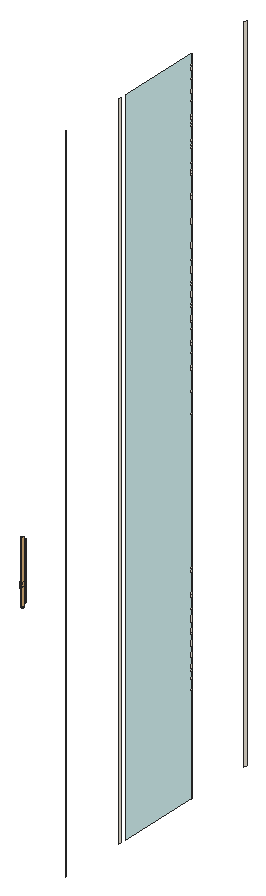
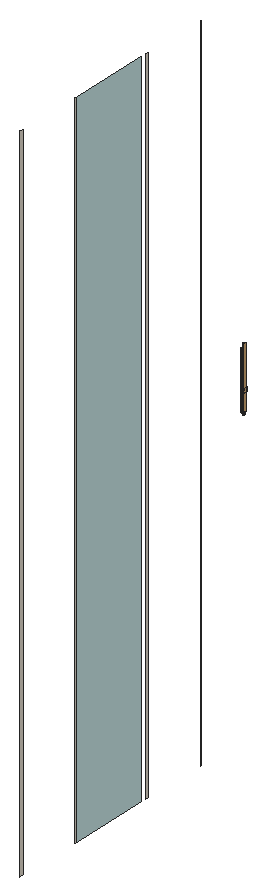
# SketchUp Ruby script. Lengths in inches.
U = 1.inch
M = Sketchup.active_model
def pt(a) = Geom::Point3d.new(a.map { |v| v * U })
def face(e, loops, mat)
  f = e.add_face(loops[0].map { |a| pt(a) })
  loops[1..].each { |l| e.add_face(l.map { |a| pt(a) }).erase! }
  f.material = f.back_material = mat if mat
  f
end
# faces: each face lists its corners as indices into pts; further lists are holes
def faces(e, pts, list, mat = nil) = list.each { |f| face(e, (f[0].is_a?(Array) ? f : [f]).map { |l| l.map { |i| pts[i] } }, mat) }
# xy, xz, yz: faces in a plane at the given z, y or x. An outline is a flat list of corners, or four numbers for a rectangle; further outlines are holes
def ring(l) = l.size == 4 ? [[l[0], l[1]], [l[2], l[1]], [l[2], l[3]], [l[0], l[3]]] : l.each_slice(2).to_a
def flat(e, list, mat, &to3) = list.each { |f| face(e, (f[0].is_a?(Array) ? f : [f]).map { |l| ring(l).map { |u, v| to3.(u, v) } }, mat) }
def xy(e, z, list, mat = nil) = flat(e, list, mat) { |x, y| [x, y, z] }
def xz(e, y, list, mat = nil) = flat(e, list, mat) { |x, z| [x, y, z] }
def yz(e, x, list, mat = nil) = flat(e, list, mat) { |y, z| [x, y, z] }
def lines(e, pts, list) = list.each { |a, b| e.add_line(pt(pts[a]), pt(pts[b])) }
# prism: a flat outline (further loops are holes) pulled along v
def prism(e, loops, v, mat = nil)
  f = face(e, loops, mat); d = Geom::Vector3d.new(v.map { |x| x * U })
  f.pushpull(f.normal.samedirection?(d) ? d.length : -d.length)
end
def box(e, o, s, mat = nil) = prism(e, [[o, [o[0] + s[0], o[1], o[2]], [o[0] + s[0], o[1] + s[1], o[2]], [o[0], o[1] + s[1], o[2]]]], [0, 0, s[2]], mat)
def at(x, y, z, deg = 0) = Geom::Transformation.translation(pt([x, y, z])) * Geom::Transformation.rotation(ORIGIN, Z_AXIS, deg.degrees)
def axes(o, x, y, z) = Geom::Transformation.new([*x, 0, *y, 0, *z, 0, *pt(o).to_a, 1])
def part(name) = M.definitions.add(name)
# library, detail: a bought-in or finely detailed component or shape, given as its bounding box
def library(name, o, s) = part(name).tap { |d| box(d.entities, o, s) }
def detail(e, o, s) = box(e.add_group.entities, o, s)
def put(e, d, t, mat = nil) = e.add_instance(d, t).tap { |i| i.material = mat if mat }
def group(e, t, mat = nil) = e.add_group.tap { |g| g.transformation = t; g.material = mat if mat }.entities
root = M.entities
M.materials.add("Material \#1").color = [140, 140, 140]
M.materials.add("[0030_OldLace]").color = [253, 245, 230]
M.materials.add("[0090_LightCyan]").color = [224, 255, 255]
c1 = library("3DGeom~1_Defintion",[-60.87,347.29,-704.08],[121.74,121.75,1000])
c2 = library("3DGeom~14_Defintion",[-102.17,352.37,-727.27],[204.35,204.35,1000])
c3 = part("3DGeom~5_Defintion")
xy(c3.entities,-225.24,[[-0.79,-499.98,-2.33,-499.64,7.45,-496.14],[-0.79,-499.98,7.45,-496.14,1.58,-499.88],[1.58,-499.88,7.45,-496.14,3.84,-499.16],[-2.33,-499.64,7.4,-485.75,7.45,-496.14],[3.84,-499.16,7.45,-496.14,5.85,-497.89],
  [7.45,-496.14,7.4,-485.75,8.24,-487.08],[7.45,-496.14,8.24,-487.08,8.96,-489.34],[7.45,-496.14,8.96,-489.34,9.0625,-491.71],[7.45,-496.14,9.0625,-491.71,8.55,-494.03],[-7.4,-496.08,-8.24,-494.76,2.32,-482.2],
  [-8.24,-494.76,-8.96,-492.5,2.32,-482.2],[-8.96,-492.5,-9.0625,-490.125,2.32,-482.2],[-9.0625,-490.125,-8.55,-487.81,2.32,-482.2],[-8.55,-487.81,-7.45,-485.7,2.32,-482.2],[-7.45,-485.7,-5.85,-483.95,2.32,-482.2],
  [-5.85,-483.95,-3.84,-482.68,2.32,-482.2],[-3.84,-482.68,-1.58,-481.96,2.32,-482.2],[2.32,-482.2,-1.58,-481.96,0.79,-481.86],[0,481.82,-2.35,482.13,-6.92,496.71],[0,481.82,-6.92,496.71,1.55,482.04],
  [-2.35,482.13,-4.55,483.04,-6.92,496.71],[-4.55,483.04,-6.43,484.49,-6.92,496.71],[-6.43,484.49,-7.88,486.37,-6.92,496.71],[6.92,485.12,-1.55,499.8125,7.88,495.47],[6.92,485.12,7.88,495.47,7.88,486.37],
  [-7.88,486.37,-8.79,488.57,-6.92,496.71],[7.88,486.37,7.88,495.47,8.79,488.57],[-8.79,488.57,-9.1,490.92,-6.92,496.71],[8.79,488.57,7.88,495.47,9.1,490.92],[-9.1,490.92,-8.79,493.28,-6.92,496.71],
  [9.1,490.92,7.88,495.47,8.79,493.28],[-8.79,493.28,-7.88,495.47,-6.92,496.71],[7.88,495.47,-1.55,499.8125,0,500.02],[7.88,495.47,0,500.02,2.35,499.71],[7.88,495.47,2.35,499.71,4.55,498.8],
  [7.88,495.47,4.55,498.8,6.43,497.35]],"Material \#1")
xy(c3.entities,-221.57,[[-2.33,-499.64,-5.22,-498.37,7.4,-485.75],[-5.22,-498.37,-7.4,-496.08,5.22,-483.47],[-5.22,-498.37,5.22,-483.47,7.4,-485.75],[-7.4,-496.08,2.32,-482.2,5.22,-483.47],[1.55,482.04,-6.92,496.71,-4.55,498.8],
  [1.55,482.04,-4.55,498.8,4.55,483.04],[4.55,483.04,-4.55,498.8,-1.55,499.8125],[4.55,483.04,-1.55,499.8125,6.92,485.12]],"Material \#1")
xy(c3.entities,38.05,[[-2.33,-499.64,7.4,-485.75,-5.22,-498.37],[-5.22,-498.37,5.22,-483.47,-7.4,-496.08],[-5.22,-498.37,7.4,-485.75,5.22,-483.47],[-7.4,-496.08,5.22,-483.47,2.32,-482.2],[1.55,482.04,-4.55,498.8,-6.92,496.71],
  [1.55,482.04,4.55,483.04,-4.55,498.8],[4.55,483.04,-1.55,499.8125,-4.55,498.8],[4.55,483.04,6.92,485.12,-1.55,499.8125]],"Material \#1")
xy(c3.entities,41.72,[[-0.79,-499.98,7.45,-496.14,-2.33,-499.64],[-0.79,-499.98,1.58,-499.88,7.45,-496.14],[1.58,-499.88,3.84,-499.16,7.45,-496.14],[-2.33,-499.64,7.45,-496.14,7.4,-485.75],[3.84,-499.16,5.85,-497.89,7.45,-496.14],
  [7.45,-496.14,8.24,-487.08,7.4,-485.75],[7.45,-496.14,8.55,-494.03,9.0625,-491.71],[7.45,-496.14,8.96,-489.34,8.24,-487.08],[7.45,-496.14,9.0625,-491.71,8.96,-489.34],[-7.4,-496.08,2.32,-482.2,-8.24,-494.76],
  [-8.24,-494.76,2.32,-482.2,-8.96,-492.5],[-8.96,-492.5,2.32,-482.2,-9.0625,-490.125],[-9.0625,-490.125,2.32,-482.2,-8.55,-487.81],[-8.55,-487.81,2.32,-482.2,-7.45,-485.7],[-7.45,-485.7,2.32,-482.2,-5.85,-483.95],
  [-5.85,-483.95,2.32,-482.2,-3.84,-482.68],[-3.84,-482.68,2.32,-482.2,-1.58,-481.96],[2.32,-482.2,0.79,-481.86,-1.58,-481.96],[0,481.82,-6.92,496.71,-2.35,482.13],[0,481.82,1.55,482.04,-6.92,496.71],
  [-2.35,482.13,-6.92,496.71,-4.55,483.04],[-4.55,483.04,-6.92,496.71,-6.43,484.49],[-6.43,484.49,-6.92,496.71,-7.88,486.37],[6.92,485.12,7.88,495.47,-1.55,499.8125],[6.92,485.12,7.88,486.37,7.88,495.47],
  [-7.88,486.37,-6.92,496.71,-8.79,488.57],[7.88,486.37,8.79,488.57,7.88,495.47],[-8.79,488.57,-6.92,496.71,-9.1,490.92],[8.79,488.57,9.1,490.92,7.88,495.47],[-9.1,490.92,-6.92,496.71,-8.79,493.28],
  [9.1,490.92,8.79,493.28,7.88,495.47],[-8.79,493.28,-6.92,496.71,-7.88,495.47],[7.88,495.47,0,500.02,-1.55,499.8125],[7.88,495.47,2.35,499.71,0,500.02],[7.88,495.47,4.55,498.8,2.35,499.71],
  [7.88,495.47,6.43,497.35,4.55,498.8]],"Material \#1")
c4 = library("3DGeom~4_Defintion",[-18.02,-499.97,-221.16],[36.04,1000,262.12])
yz(root,153,[[457.1,0,457.147,120],[469.008,0,469.475,120],[485.35,0,485.397,120],[497.258,0,497.725,120]],"[0030_OldLace]")
yz(root,153,[[470.555,0,485.35,120]],"[0090_LightCyan]")
yz(root,155.637,[[444.023,49.872,444.023,49.887,443.91,49.886],[444.023,49.872,444.135,49.901,444.023,49.887],[444.023,49.872,444.137,49.886,444.135,49.901],[444.137,49.886,444.239,49.941,444.135,49.901],[444.137,49.886,444.243,49.927,444.239,49.941],
  [444.243,49.927,444.336,50.005,444.239,49.941],[444.243,49.927,444.341,49.992,444.336,50.005],[444.341,49.992,444.422,50.09,444.336,50.005],[444.341,49.992,444.429,50.078,444.422,50.09],[444.429,50.078,444.494,50.19,444.422,50.09],
  [444.429,50.078,444.503,50.18,444.494,50.19],[444.023,50.107,444.023,50.122,443.986,50.111],[444.023,50.107,444.059,50.126,444.023,50.122],[444.023,50.107,444.061,50.111,444.059,50.126],[443.986,50.111,443.988,50.126,443.95,50.125],
  [443.986,50.111,444.023,50.122,443.988,50.126],[444.061,50.111,444.092,50.139,444.059,50.126],[444.061,50.111,444.096,50.125,444.092,50.139],[443.95,50.125,443.988,50.126,443.954,50.139],[444.096,50.125,444.123,50.16,444.092,50.139],
  [444.096,50.125,444.129,50.147,444.123,50.16],[444.129,50.147,444.151,50.187,444.123,50.16],[444.129,50.147,444.158,50.175,444.151,50.187],[444.158,50.175,444.175,50.22,444.151,50.187],[444.158,50.175,444.183,50.211,444.175,50.22],
  [444.503,50.18,444.558,50.315,444.494,50.19],[444.503,50.18,444.568,50.307,444.558,50.315],[444.183,50.211,444.195,50.259,444.175,50.22],[444.183,50.211,444.204,50.251,444.195,50.259],[444.204,50.251,444.209,50.302,444.195,50.259],
  [444.204,50.251,444.22,50.297,444.209,50.302],[444.22,50.297,444.219,50.349,444.209,50.302],[444.22,50.297,444.229,50.346,444.219,50.349],[444.568,50.307,444.604,50.449,444.558,50.315],[444.568,50.307,444.614,50.444,444.604,50.449],
  [444.229,50.346,444.222,50.385,444.219,50.349],[444.229,50.346,444.233,50.385,444.222,50.385],[444.222,50.385,444.233,50.385,444.219,50.448],[444.233,50.385,444.229,50.451,444.219,50.448],[444.614,50.444,444.633,50.595,444.604,50.449],
  [444.614,50.444,444.644,50.592,444.633,50.595],[444.219,50.448,444.229,50.451,444.209,50.495],[444.229,50.451,444.22,50.5,444.209,50.495],[444.209,50.495,444.22,50.5,444.195,50.538],[444.22,50.5,444.204,50.546,444.195,50.538],
  [444.195,50.538,444.204,50.546,444.175,50.577],[444.204,50.546,444.183,50.587,444.175,50.577],[444.175,50.577,444.183,50.587,444.151,50.61],[444.183,50.587,444.158,50.622,444.151,50.61],[444.644,50.592,444.643,50.757,444.633,50.595],
  [444.644,50.592,444.654,50.756,444.643,50.757],[444.151,50.61,444.158,50.622,444.123,50.637],[444.158,50.622,444.129,50.651,444.123,50.637],[444.123,50.637,444.129,50.651,444.092,50.658],[444.129,50.651,444.096,50.672,444.092,50.658],
  [443.954,50.658,443.986,50.686,443.95,50.672],[443.954,50.658,443.988,50.671,443.986,50.686],[444.092,50.658,444.096,50.672,444.059,50.671],[443.988,50.671,444.023,50.69,443.986,50.686],[443.988,50.671,444.023,50.675,444.023,50.69],
  [444.059,50.671,444.061,50.686,444.023,50.675],[444.059,50.671,444.096,50.672,444.061,50.686],[444.023,50.675,444.061,50.686,444.023,50.69],[444.654,50.756,444.643,60.789,444.643,50.757],[444.654,50.756,444.654,60.79,444.643,60.789]],"Material \#1")
yz(root,155.783,[[444.137,49.886,444.135,49.901,444.239,49.941],[444.137,49.886,444.239,49.941,444.243,49.927],[444.243,49.927,444.239,49.941,444.336,50.005],[444.096,50.125,444.092,50.139,444.123,50.16],[444.096,50.125,444.123,50.16,444.129,50.147],
  [444.129,50.147,444.123,50.16,444.151,50.187],[444.129,50.147,444.151,50.187,444.158,50.175],[444.158,50.175,444.151,50.187,444.175,50.22],[444.158,50.175,444.175,50.22,444.183,50.211],[444.183,50.211,444.175,50.22,444.195,50.259],
  [444.614,50.444,444.604,50.449,444.633,50.595],[444.614,50.444,444.633,50.595,444.644,50.592],[444.129,50.651,444.092,50.658,444.096,50.672],[444.092,50.658,444.059,50.671,444.096,50.672],[443.988,50.671,443.986,50.686,444.023,50.69],
  [443.988,50.671,444.023,50.69,444.023,50.675],[444.059,50.671,444.023,50.675,444.061,50.686],[444.059,50.671,444.061,50.686,444.096,50.672],[444.023,50.675,444.023,50.69,444.061,50.686],[444.654,50.756,444.643,60.789,444.654,60.79]],"Material \#1")
p = [[155.637,444.048,50.272],[155.637,444.061,50.238],[155.639,444.061,50.238],[155.639,444.048,50.272],[155.783,444.048,50.272],[155.781,444.048,50.272],
  [155.781,444.061,50.238],[155.783,444.061,50.238],[155.637,444.084,50.251],[155.639,444.084,50.251],[155.781,444.084,50.251],[155.783,444.084,50.251],
  [155.637,444.035,50.301],[155.639,444.035,50.301],[155.637,444.078,50.335],[155.637,444.011,50.496],[155.639,444.011,50.496],[155.639,444.078,50.335],
  [155.637,443.969,50.462],[155.639,443.969,50.462],[155.783,444.035,50.301],[155.781,444.035,50.301],[155.783,444.078,50.335],[155.781,444.078,50.335],
  [155.781,444.011,50.496],[155.783,444.011,50.496],[155.783,443.969,50.462],[155.781,443.969,50.462],[155.637,444.104,50.272],[155.639,444.104,50.272],
  [155.637,444.09,50.306],[155.639,444.09,50.306],[155.781,444.104,50.272],[155.783,444.104,50.272],[155.781,444.09,50.306],[155.783,444.09,50.306],
  [155.637,443.962,50.546],[155.637,443.942,50.525],[155.639,443.942,50.525],[155.639,443.962,50.546],[155.637,443.956,50.492],[155.639,443.956,50.492],
  [155.783,443.962,50.546],[155.781,443.962,50.546],[155.781,443.942,50.525],[155.783,443.942,50.525],[155.781,443.956,50.492],[155.783,443.956,50.492],
  [155.637,443.999,50.526],[155.639,443.999,50.526],[155.637,443.985,50.559],[155.639,443.985,50.559],[155.781,443.999,50.526],[155.783,443.999,50.526],
  [155.781,443.985,50.559],[155.783,443.985,50.559]]
faces(root,p,[[0,1,2],[2,3,0],[4,5,6],[6,7,4],[1,8,9],[9,2,1],[7,6,10],[10,11,7],
  [12,0,3],[3,13,12],[14,15,16],[16,17,14],[18,12,13],[13,19,18],[20,21,5],[5,4,20],
  [22,23,24],[24,25,22],[26,27,21],[21,20,26],[8,28,29],[29,9,8],[28,30,31],[31,29,28],
  [30,14,17],[17,31,30],[11,10,32],[32,33,11],[33,32,34],[34,35,33],[35,34,23],[23,22,35],
  [36,37,38],[38,39,36],[37,40,41],[41,38,37],[42,43,44],[44,45,42],[45,44,46],[46,47,45],
  [15,48,49],[49,16,15],[48,50,51],[51,49,48],[50,36,39],[39,51,50],[40,18,19],[19,41,40],
  [25,24,52],[52,53,25],[53,52,54],[54,55,53],[55,54,43],[43,42,55],[47,46,27],[27,26,47]],"Material \#1")
put(root,c1,axes([155.66,444.02,55.77],[0,-0.00353,0],[0,0,-0.00492],[-0.00025,0,0]),"Material \#1")
put(root,c2,axes([155.66,444.02,55.77],[0,-0.00317,0],[0,0,-0.00442],[-0.00022,0,0]),"Material \#1")
put(root,c3,axes([155.66,444.02,55.77],[0,-0.00786,0],[0,0,-0.01095],[-0.00055,0,0]),"Material \#1")
put(root,c4,axes([155.66,444.02,55.77],[0,-0.008,0],[0,0,-0.01115],[-0.00056,0,0]),"Material \#1")
